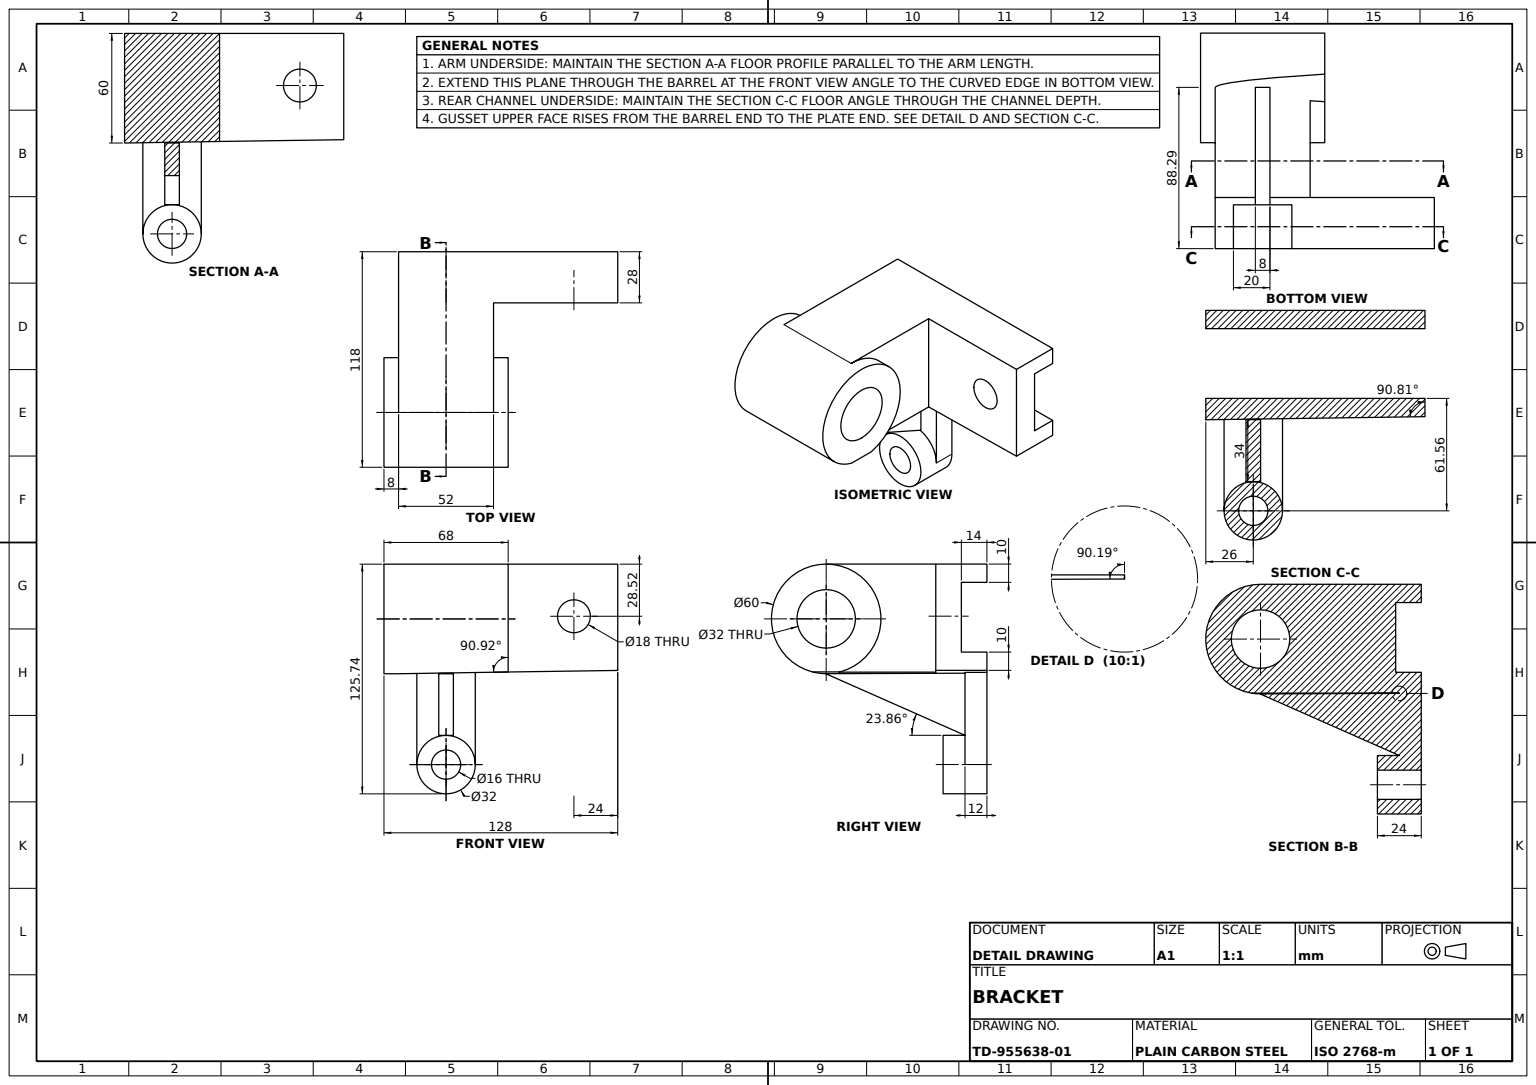
ISO-10303-21;
HEADER;
FILE_DESCRIPTION((''),'2;1');
FILE_NAME('','',(''),(''),'','','');
FILE_SCHEMA(('AUTOMOTIVE_DESIGN'));
ENDSEC;
DATA;
#1=APPLICATION_CONTEXT('');
#2=PRODUCT_CONTEXT('',#1,'mechanical');
#3=PRODUCT('','','',(#2));
#4=PRODUCT_DEFINITION_FORMATION('','',#3);
#5=PRODUCT_DEFINITION_CONTEXT('',#1,'design');
#6=PRODUCT_DEFINITION('','',#4,#5);
#7=PRODUCT_DEFINITION_SHAPE('','',#6);
#8=(LENGTH_UNIT()NAMED_UNIT(*)SI_UNIT(.MILLI.,.METRE.));
#9=(NAMED_UNIT(*)PLANE_ANGLE_UNIT()SI_UNIT($,.RADIAN.));
#10=(NAMED_UNIT(*)SI_UNIT($,.STERADIAN.)SOLID_ANGLE_UNIT());
#11=UNCERTAINTY_MEASURE_WITH_UNIT(LENGTH_MEASURE(1.E-05),#8,'distance_accuracy_value','');
#12=(GEOMETRIC_REPRESENTATION_CONTEXT(3)GLOBAL_UNCERTAINTY_ASSIGNED_CONTEXT((#11))GLOBAL_UNIT_ASSIGNED_CONTEXT((#8,#9,#10))REPRESENTATION_CONTEXT('',''));
#13=CARTESIAN_POINT('',(113.,31.478195,14.));
#14=VERTEX_POINT('',#13);
#15=CARTESIAN_POINT('',(113.,31.478195,28.));
#16=VERTEX_POINT('',#15);
#17=CARTESIAN_POINT('',(113.,31.478195,-100.));
#18=DIRECTION('',(0.,0.,1.));
#19=VECTOR('',#18,1000.);
#20=LINE('',#17,#19);
#21=EDGE_CURVE('',#14,#16,#20,.T.);
#22=ORIENTED_EDGE('',*,*,#21,.T.);
#23=CARTESIAN_POINT('',(95.,31.478195,28.));
#24=VERTEX_POINT('',#23);
#25=CARTESIAN_POINT('',(104.,31.478195,28.));
#26=DIRECTION('',(1.,0.,0.));
#27=AXIS2_PLACEMENT_3D('',#25,#18,#26);
#28=CIRCLE('',#27,9.);
#29=EDGE_CURVE('',#16,#24,#28,.T.);
#30=ORIENTED_EDGE('',*,*,#29,.T.);
#31=CARTESIAN_POINT('',(95.,31.478195,14.));
#32=VERTEX_POINT('',#31);
#33=CARTESIAN_POINT('',(95.,31.478195,-100.));
#34=LINE('',#33,#19);
#35=EDGE_CURVE('',#32,#24,#34,.T.);
#36=ORIENTED_EDGE('',*,*,#35,.F.);
#37=CARTESIAN_POINT('',(104.,31.478195,14.));
#38=AXIS2_PLACEMENT_3D('',#37,#18,#26);
#39=CIRCLE('',#38,9.);
#40=EDGE_CURVE('',#14,#32,#39,.T.);
#41=ORIENTED_EDGE('',*,*,#40,.F.);
#42=EDGE_LOOP('',(#22,#30,#36,#41));
#43=FACE_OUTER_BOUND('',#42,.T.);
#44=CARTESIAN_POINT('',(104.,31.478195,-100.));
#45=AXIS2_PLACEMENT_3D('',#44,#18,#26);
#46=CYLINDRICAL_SURFACE('',#45,9.);
#47=ADVANCED_FACE('',(#43),#46,.F.);
#48=CARTESIAN_POINT('',(50.,-49.744681,24.));
#49=VERTEX_POINT('',#48);
#50=CARTESIAN_POINT('',(50.,-49.744681,12.));
#51=VERTEX_POINT('',#50);
#52=DIRECTION('',(0.,0.,-1.));
#53=VECTOR('',#52,1000.);
#54=LINE('',#50,#53);
#55=EDGE_CURVE('',#49,#51,#54,.T.);
#56=ORIENTED_EDGE('',*,*,#55,.T.);
#57=CARTESIAN_POINT('',(34.,-33.744681,12.));
#58=VERTEX_POINT('',#57);
#59=CARTESIAN_POINT('',(34.,-49.744681,12.));
#60=AXIS2_PLACEMENT_3D('',#59,#18,#26);
#61=CIRCLE('',#60,16.);
#62=EDGE_CURVE('',#51,#58,#61,.T.);
#63=ORIENTED_EDGE('',*,*,#62,.T.);
#64=CARTESIAN_POINT('',(18.,-49.744681,12.));
#65=VERTEX_POINT('',#64);
#66=EDGE_CURVE('',#58,#65,#61,.T.);
#67=ORIENTED_EDGE('',*,*,#66,.T.);
#68=CARTESIAN_POINT('',(18.,-49.744681,24.));
#69=VERTEX_POINT('',#68);
#70=LINE('',#64,#53);
#71=EDGE_CURVE('',#69,#65,#70,.T.);
#72=ORIENTED_EDGE('',*,*,#71,.F.);
#73=CARTESIAN_POINT('',(34.,-49.744681,24.));
#74=AXIS2_PLACEMENT_3D('',#73,#18,#26);
#75=CIRCLE('',#74,16.);
#76=EDGE_CURVE('',#49,#69,#75,.T.);
#77=ORIENTED_EDGE('',*,*,#76,.F.);
#78=EDGE_LOOP('',(#56,#63,#67,#72,#77));
#79=FACE_OUTER_BOUND('',#78,.T.);
#80=DIRECTION('',(-1.,0.,0.));
#81=AXIS2_PLACEMENT_3D('',#59,#52,#80);
#82=CYLINDRICAL_SURFACE('',#81,16.);
#83=ADVANCED_FACE('',(#79),#82,.T.);
#84=CARTESIAN_POINT('',(8.,0.113475,28.));
#85=VERTEX_POINT('',#84);
#86=CARTESIAN_POINT('',(60.,0.851064,28.));
#87=VERTEX_POINT('',#86);
#88=CARTESIAN_POINT('',(0.,0.,28.));
#89=DIRECTION('',(0.999899417,0.01418297,0.));
#90=VECTOR('',#89,1000.);
#91=LINE('',#88,#90);
#92=EDGE_CURVE('',#85,#87,#91,.T.);
#93=ORIENTED_EDGE('',*,*,#92,.T.);
#94=CARTESIAN_POINT('',(60.,0.835934,28.));
#95=VERTEX_POINT('',#94);
#96=CARTESIAN_POINT('',(60.,60.,28.));
#97=DIRECTION('',(0.,1.,0.));
#98=VECTOR('',#97,1000.);
#99=LINE('',#96,#98);
#100=EDGE_CURVE('',#95,#87,#99,.T.);
#101=ORIENTED_EDGE('',*,*,#100,.F.);
#102=CARTESIAN_POINT('',(8.,0.,28.));
#103=VERTEX_POINT('',#102);
#104=CARTESIAN_POINT('',(68.,0.964539,28.));
#105=DIRECTION('',(0.999870812,0.016073573,0.));
#106=VECTOR('',#105,1000.);
#107=LINE('',#104,#106);
#108=EDGE_CURVE('',#103,#95,#107,.T.);
#109=ORIENTED_EDGE('',*,*,#108,.F.);
#110=LINE('',#102,#98);
#111=EDGE_CURVE('',#103,#85,#110,.T.);
#112=ORIENTED_EDGE('',*,*,#111,.T.);
#113=EDGE_LOOP('',(#93,#101,#109,#112));
#114=FACE_OUTER_BOUND('',#113,.T.);
#115=CARTESIAN_POINT('',(68.,0.,28.));
#116=AXIS2_PLACEMENT_3D('',#115,#52,#80);
#117=PLANE('',#116);
#118=ADVANCED_FACE('',(#114),#117,.T.);
#119=CARTESIAN_POINT('',(8.,11.815603,0.));
#120=VERTEX_POINT('',#119);
#121=CARTESIAN_POINT('',(8.,0.113475,0.));
#122=VERTEX_POINT('',#121);
#123=DIRECTION('',(0.,-1.,0.));
#124=VECTOR('',#123,1000.);
#125=LINE('',#119,#124);
#126=EDGE_CURVE('',#120,#122,#125,.T.);
#127=ORIENTED_EDGE('',*,*,#126,.T.);
#128=LINE('',#84,#19);
#129=EDGE_CURVE('',#122,#85,#128,.T.);
#130=ORIENTED_EDGE('',*,*,#129,.T.);
#131=ORIENTED_EDGE('',*,*,#111,.F.);
#132=CARTESIAN_POINT('',(8.,0.,88.));
#133=VERTEX_POINT('',#132);
#134=CARTESIAN_POINT('',(8.,0.,0.));
#135=LINE('',#134,#19);
#136=EDGE_CURVE('',#103,#133,#135,.T.);
#137=ORIENTED_EDGE('',*,*,#136,.T.);
#138=CARTESIAN_POINT('',(8.,60.,88.));
#139=VERTEX_POINT('',#138);
#140=CARTESIAN_POINT('',(8.,30.,88.));
#141=AXIS2_PLACEMENT_3D('',#140,#26,#123);
#142=CIRCLE('',#141,30.);
#143=EDGE_CURVE('',#133,#139,#142,.T.);
#144=ORIENTED_EDGE('',*,*,#143,.T.);
#145=CARTESIAN_POINT('',(8.,60.,0.));
#146=VERTEX_POINT('',#145);
#147=LINE('',#145,#53);
#148=EDGE_CURVE('',#139,#146,#147,.T.);
#149=ORIENTED_EDGE('',*,*,#148,.T.);
#150=CARTESIAN_POINT('',(8.,50.,0.));
#151=VERTEX_POINT('',#150);
#152=LINE('',#145,#124);
#153=EDGE_CURVE('',#146,#151,#152,.T.);
#154=ORIENTED_EDGE('',*,*,#153,.T.);
#155=CARTESIAN_POINT('',(8.,50.,14.));
#156=VERTEX_POINT('',#155);
#157=LINE('',#150,#19);
#158=EDGE_CURVE('',#151,#156,#157,.T.);
#159=ORIENTED_EDGE('',*,*,#158,.T.);
#160=CARTESIAN_POINT('',(8.,11.815603,14.));
#161=VERTEX_POINT('',#160);
#162=LINE('',#155,#124);
#163=EDGE_CURVE('',#156,#161,#162,.T.);
#164=ORIENTED_EDGE('',*,*,#163,.T.);
#165=LINE('',#160,#53);
#166=EDGE_CURVE('',#161,#120,#165,.T.);
#167=ORIENTED_EDGE('',*,*,#166,.T.);
#168=EDGE_LOOP('',(#127,#130,#131,#137,#144,#149,#154,#159,#164,#167));
#169=FACE_OUTER_BOUND('',#168,.T.);
#170=AXIS2_PLACEMENT_3D('',#140,#80,#123);
#171=PLANE('',#170);
#172=ADVANCED_FACE('',(#169),#171,.T.);
#173=CARTESIAN_POINT('',(0.,60.,88.));
#174=VERTEX_POINT('',#173);
#175=VECTOR('',#26,1000.);
#176=LINE('',#173,#175);
#177=EDGE_CURVE('',#174,#139,#176,.T.);
#178=ORIENTED_EDGE('',*,*,#177,.F.);
#179=CARTESIAN_POINT('',(0.,0.,88.));
#180=VERTEX_POINT('',#179);
#181=CARTESIAN_POINT('',(0.,30.,88.));
#182=AXIS2_PLACEMENT_3D('',#181,#26,#97);
#183=CIRCLE('',#182,30.);
#184=EDGE_CURVE('',#174,#180,#183,.T.);
#185=ORIENTED_EDGE('',*,*,#184,.T.);
#186=LINE('',#179,#175);
#187=EDGE_CURVE('',#180,#133,#186,.T.);
#188=ORIENTED_EDGE('',*,*,#187,.T.);
#189=CARTESIAN_POINT('',(68.,0.964539,95.545993));
#190=VERTEX_POINT('',#189);
#191=CARTESIAN_POINT('',(28.108187,0.323252,93.07845));
#192=CARTESIAN_POINT('',(8.,0.,90.549513));
#193=(BOUNDED_CURVE()B_SPLINE_CURVE(3,(#189,#191,#192,#132),.UNSPECIFIED.,.F.,.F.)B_SPLINE_CURVE_WITH_KNOTS((4,4),(2.887328708,3.141592654),.UNSPECIFIED.)CURVE()GEOMETRIC_REPRESENTATION_ITEM()RATIONAL_B_SPLINE_CURVE((1.,0.99461974,0.99461974,1.))REPRESENTATION_ITEM(''));
#194=EDGE_CURVE('',#190,#133,#193,.T.);
#195=ORIENTED_EDGE('',*,*,#194,.F.);
#196=CARTESIAN_POINT('',(68.,60.,88.));
#197=VERTEX_POINT('',#196);
#198=CARTESIAN_POINT('',(68.,30.,88.));
#199=AXIS2_PLACEMENT_3D('',#198,#26,#97);
#200=CIRCLE('',#199,30.);
#201=EDGE_CURVE('',#197,#190,#200,.T.);
#202=ORIENTED_EDGE('',*,*,#201,.F.);
#203=CARTESIAN_POINT('',(60.,60.,88.));
#204=VERTEX_POINT('',#203);
#205=EDGE_CURVE('',#204,#197,#176,.T.);
#206=ORIENTED_EDGE('',*,*,#205,.F.);
#207=VECTOR('',#80,1000.);
#208=LINE('',#196,#207);
#209=EDGE_CURVE('',#204,#139,#208,.T.);
#210=ORIENTED_EDGE('',*,*,#209,.T.);
#211=EDGE_LOOP('',(#178,#185,#188,#195,#202,#206,#210));
#212=FACE_OUTER_BOUND('',#211,.T.);
#213=CYLINDRICAL_SURFACE('',#182,30.);
#214=ADVANCED_FACE('',(#212),#213,.T.);
#215=CARTESIAN_POINT('',(18.,0.255319,12.));
#216=VERTEX_POINT('',#215);
#217=CARTESIAN_POINT('',(18.,0.255319,0.));
#218=VERTEX_POINT('',#217);
#219=LINE('',#215,#53);
#220=EDGE_CURVE('',#216,#218,#219,.T.);
#221=ORIENTED_EDGE('',*,*,#220,.T.);
#222=CARTESIAN_POINT('',(18.,-49.744681,0.));
#223=VERTEX_POINT('',#222);
#224=LINE('',#217,#98);
#225=EDGE_CURVE('',#223,#218,#224,.T.);
#226=ORIENTED_EDGE('',*,*,#225,.F.);
#227=EDGE_CURVE('',#65,#223,#70,.T.);
#228=ORIENTED_EDGE('',*,*,#227,.F.);
#229=LINE('',#215,#98);
#230=EDGE_CURVE('',#65,#216,#229,.T.);
#231=ORIENTED_EDGE('',*,*,#230,.T.);
#232=EDGE_LOOP('',(#221,#226,#228,#231));
#233=FACE_OUTER_BOUND('',#232,.T.);
#234=AXIS2_PLACEMENT_3D('',#215,#80,#123);
#235=PLANE('',#234);
#236=ADVANCED_FACE('',(#233),#235,.T.);
#237=CARTESIAN_POINT('',(42.,-49.744681,0.));
#238=VERTEX_POINT('',#237);
#239=CARTESIAN_POINT('',(42.,-49.744681,24.));
#240=VERTEX_POINT('',#239);
#241=LINE('',#237,#19);
#242=EDGE_CURVE('',#238,#240,#241,.T.);
#243=ORIENTED_EDGE('',*,*,#242,.F.);
#244=CARTESIAN_POINT('',(26.,-49.744681,0.));
#245=VERTEX_POINT('',#244);
#246=CARTESIAN_POINT('',(34.,-49.744681,0.));
#247=AXIS2_PLACEMENT_3D('',#246,#18,#26);
#248=CIRCLE('',#247,8.);
#249=EDGE_CURVE('',#245,#238,#248,.T.);
#250=ORIENTED_EDGE('',*,*,#249,.F.);
#251=CARTESIAN_POINT('',(26.,-49.744681,24.));
#252=VERTEX_POINT('',#251);
#253=LINE('',#244,#19);
#254=EDGE_CURVE('',#245,#252,#253,.T.);
#255=ORIENTED_EDGE('',*,*,#254,.T.);
#256=CIRCLE('',#74,8.);
#257=EDGE_CURVE('',#252,#240,#256,.T.);
#258=ORIENTED_EDGE('',*,*,#257,.T.);
#259=EDGE_LOOP('',(#243,#250,#255,#258));
#260=FACE_OUTER_BOUND('',#259,.T.);
#261=CYLINDRICAL_SURFACE('',#247,8.);
#262=ADVANCED_FACE('',(#260),#261,.F.);
#263=CARTESIAN_POINT('',(0.,46.,88.));
#264=VERTEX_POINT('',#263);
#265=CARTESIAN_POINT('',(68.,46.,88.));
#266=VERTEX_POINT('',#265);
#267=LINE('',#263,#175);
#268=EDGE_CURVE('',#264,#266,#267,.T.);
#269=ORIENTED_EDGE('',*,*,#268,.F.);
#270=CARTESIAN_POINT('',(0.,14.,88.));
#271=VERTEX_POINT('',#270);
#272=CIRCLE('',#182,16.);
#273=EDGE_CURVE('',#271,#264,#272,.T.);
#274=ORIENTED_EDGE('',*,*,#273,.F.);
#275=CARTESIAN_POINT('',(68.,14.,88.));
#276=VERTEX_POINT('',#275);
#277=LINE('',#270,#175);
#278=EDGE_CURVE('',#271,#276,#277,.T.);
#279=ORIENTED_EDGE('',*,*,#278,.T.);
#280=CIRCLE('',#199,16.);
#281=EDGE_CURVE('',#276,#266,#280,.T.);
#282=ORIENTED_EDGE('',*,*,#281,.T.);
#283=EDGE_LOOP('',(#269,#274,#279,#282));
#284=FACE_OUTER_BOUND('',#283,.T.);
#285=CYLINDRICAL_SURFACE('',#182,16.);
#286=ADVANCED_FACE('',(#284),#285,.F.);
#287=CARTESIAN_POINT('',(50.,0.70922,0.));
#288=VERTEX_POINT('',#287);
#289=CARTESIAN_POINT('',(50.,-49.744681,0.));
#290=VERTEX_POINT('',#289);
#291=LINE('',#289,#124);
#292=EDGE_CURVE('',#288,#290,#291,.T.);
#293=ORIENTED_EDGE('',*,*,#292,.T.);
#294=AXIS2_PLACEMENT_3D('',#246,#52,#80);
#295=CIRCLE('',#294,16.);
#296=EDGE_CURVE('',#290,#223,#295,.T.);
#297=ORIENTED_EDGE('',*,*,#296,.T.);
#298=ORIENTED_EDGE('',*,*,#225,.T.);
#299=CARTESIAN_POINT('',(0.,0.,0.));
#300=LINE('',#299,#90);
#301=EDGE_CURVE('',#122,#218,#300,.T.);
#302=ORIENTED_EDGE('',*,*,#301,.F.);
#303=ORIENTED_EDGE('',*,*,#126,.F.);
#304=CARTESIAN_POINT('',(128.,11.815603,0.));
#305=VERTEX_POINT('',#304);
#306=CARTESIAN_POINT('',(0.,11.815603,0.));
#307=LINE('',#306,#175);
#308=EDGE_CURVE('',#120,#305,#307,.T.);
#309=ORIENTED_EDGE('',*,*,#308,.T.);
#310=CARTESIAN_POINT('',(128.,1.815603,0.));
#311=VERTEX_POINT('',#310);
#312=LINE('',#310,#98);
#313=EDGE_CURVE('',#311,#305,#312,.T.);
#314=ORIENTED_EDGE('',*,*,#313,.F.);
#315=EDGE_CURVE('',#288,#311,#300,.T.);
#316=ORIENTED_EDGE('',*,*,#315,.F.);
#317=EDGE_LOOP('',(#293,#297,#298,#302,#303,#309,#314,#316));
#318=FACE_OUTER_BOUND('',#317,.T.);
#319=ORIENTED_EDGE('',*,*,#249,.T.);
#320=EDGE_CURVE('',#238,#245,#248,.T.);
#321=ORIENTED_EDGE('',*,*,#320,.T.);
#322=EDGE_LOOP('',(#319,#321));
#323=FACE_BOUND('',#322,.T.);
#324=AXIS2_PLACEMENT_3D('',#299,#52,#80);
#325=PLANE('',#324);
#326=ADVANCED_FACE('',(#318,#323),#325,.T.);
#327=EDGE_CURVE('',#240,#252,#256,.T.);
#328=ORIENTED_EDGE('',*,*,#327,.T.);
#329=ORIENTED_EDGE('',*,*,#254,.F.);
#330=ORIENTED_EDGE('',*,*,#320,.F.);
#331=ORIENTED_EDGE('',*,*,#242,.T.);
#332=EDGE_LOOP('',(#328,#329,#330,#331));
#333=FACE_OUTER_BOUND('',#332,.T.);
#334=ADVANCED_FACE('',(#333),#261,.F.);
#335=ORIENTED_EDGE('',*,*,#177,.T.);
#336=ORIENTED_EDGE('',*,*,#143,.F.);
#337=ORIENTED_EDGE('',*,*,#187,.F.);
#338=EDGE_CURVE('',#180,#174,#183,.T.);
#339=ORIENTED_EDGE('',*,*,#338,.T.);
#340=EDGE_LOOP('',(#335,#336,#337,#339));
#341=FACE_OUTER_BOUND('',#340,.T.);
#342=ADVANCED_FACE('',(#341),#213,.T.);
#343=EDGE_CURVE('',#51,#290,#54,.T.);
#344=ORIENTED_EDGE('',*,*,#343,.T.);
#345=ORIENTED_EDGE('',*,*,#292,.F.);
#346=CARTESIAN_POINT('',(50.,0.70922,12.));
#347=VERTEX_POINT('',#346);
#348=LINE('',#346,#53);
#349=EDGE_CURVE('',#347,#288,#348,.T.);
#350=ORIENTED_EDGE('',*,*,#349,.F.);
#351=LINE('',#50,#124);
#352=EDGE_CURVE('',#347,#51,#351,.T.);
#353=ORIENTED_EDGE('',*,*,#352,.T.);
#354=EDGE_LOOP('',(#344,#345,#350,#353));
#355=FACE_OUTER_BOUND('',#354,.T.);
#356=AXIS2_PLACEMENT_3D('',#50,#26,#97);
#357=PLANE('',#356);
#358=ADVANCED_FACE('',(#355),#357,.T.);
#359=CARTESIAN_POINT('',(38.,0.,88.292467));
#360=VERTEX_POINT('',#359);
#361=CARTESIAN_POINT('',(38.,-33.744681,12.));
#362=VERTEX_POINT('',#361);
#363=DIRECTION('',(0.,-0.404505371,-0.914535622));
#364=VECTOR('',#363,1000.);
#365=LINE('',#361,#364);
#366=EDGE_CURVE('',#360,#362,#365,.T.);
#367=ORIENTED_EDGE('',*,*,#366,.F.);
#368=CARTESIAN_POINT('',(30.,0.,88.292467));
#369=VERTEX_POINT('',#368);
#370=LINE('',#368,#175);
#371=EDGE_CURVE('',#369,#360,#370,.T.);
#372=ORIENTED_EDGE('',*,*,#371,.F.);
#373=CARTESIAN_POINT('',(30.,-33.744681,12.));
#374=VERTEX_POINT('',#373);
#375=LINE('',#373,#364);
#376=EDGE_CURVE('',#369,#374,#375,.T.);
#377=ORIENTED_EDGE('',*,*,#376,.T.);
#378=LINE('',#373,#175);
#379=EDGE_CURVE('',#374,#58,#378,.T.);
#380=ORIENTED_EDGE('',*,*,#379,.T.);
#381=LINE('',#57,#207);
#382=EDGE_CURVE('',#362,#58,#381,.T.);
#383=ORIENTED_EDGE('',*,*,#382,.F.);
#384=EDGE_LOOP('',(#367,#372,#377,#380,#383));
#385=FACE_OUTER_BOUND('',#384,.T.);
#386=DIRECTION('',(0.,-0.914535622,0.404505371));
#387=AXIS2_PLACEMENT_3D('',#373,#386,#363);
#388=PLANE('',#387);
#389=ADVANCED_FACE('',(#385),#388,.T.);
#390=ORIENTED_EDGE('',*,*,#21,.F.);
#391=EDGE_CURVE('',#32,#14,#39,.T.);
#392=ORIENTED_EDGE('',*,*,#391,.F.);
#393=ORIENTED_EDGE('',*,*,#35,.T.);
#394=EDGE_CURVE('',#24,#16,#28,.T.);
#395=ORIENTED_EDGE('',*,*,#394,.T.);
#396=EDGE_LOOP('',(#390,#392,#393,#395));
#397=FACE_OUTER_BOUND('',#396,.T.);
#398=ADVANCED_FACE('',(#397),#46,.F.);
#399=ORIENTED_EDGE('',*,*,#371,.T.);
#400=CARTESIAN_POINT('',(38.,0.255319,12.));
#401=VERTEX_POINT('',#400);
#402=DIRECTION('',(0.,-0.003346565,0.9999944));
#403=VECTOR('',#402,1000.);
#404=LINE('',#359,#403);
#405=EDGE_CURVE('',#401,#360,#404,.T.);
#406=ORIENTED_EDGE('',*,*,#405,.F.);
#407=CARTESIAN_POINT('',(30.,0.255319,12.));
#408=VERTEX_POINT('',#407);
#409=LINE('',#407,#175);
#410=EDGE_CURVE('',#408,#401,#409,.T.);
#411=ORIENTED_EDGE('',*,*,#410,.F.);
#412=LINE('',#368,#403);
#413=EDGE_CURVE('',#408,#369,#412,.T.);
#414=ORIENTED_EDGE('',*,*,#413,.T.);
#415=EDGE_LOOP('',(#399,#406,#411,#414));
#416=FACE_OUTER_BOUND('',#415,.T.);
#417=DIRECTION('',(0.,0.9999944,0.003346565));
#418=AXIS2_PLACEMENT_3D('',#368,#417,#402);
#419=PLANE('',#418);
#420=ADVANCED_FACE('',(#416),#419,.T.);
#421=CARTESIAN_POINT('',(128.,60.,28.));
#422=VERTEX_POINT('',#421);
#423=CARTESIAN_POINT('',(128.,60.,0.));
#424=VERTEX_POINT('',#423);
#425=LINE('',#421,#53);
#426=EDGE_CURVE('',#422,#424,#425,.T.);
#427=ORIENTED_EDGE('',*,*,#426,.F.);
#428=CARTESIAN_POINT('',(128.,1.815603,28.));
#429=VERTEX_POINT('',#428);
#430=LINE('',#428,#98);
#431=EDGE_CURVE('',#429,#422,#430,.T.);
#432=ORIENTED_EDGE('',*,*,#431,.F.);
#433=LINE('',#428,#53);
#434=EDGE_CURVE('',#429,#311,#433,.T.);
#435=ORIENTED_EDGE('',*,*,#434,.T.);
#436=ORIENTED_EDGE('',*,*,#313,.T.);
#437=CARTESIAN_POINT('',(128.,11.815603,14.));
#438=VERTEX_POINT('',#437);
#439=LINE('',#304,#53);
#440=EDGE_CURVE('',#438,#305,#439,.T.);
#441=ORIENTED_EDGE('',*,*,#440,.F.);
#442=CARTESIAN_POINT('',(128.,50.,14.));
#443=VERTEX_POINT('',#442);
#444=CARTESIAN_POINT('',(128.,0.,14.));
#445=LINE('',#444,#124);
#446=EDGE_CURVE('',#443,#438,#445,.T.);
#447=ORIENTED_EDGE('',*,*,#446,.F.);
#448=CARTESIAN_POINT('',(128.,50.,0.));
#449=VERTEX_POINT('',#448);
#450=LINE('',#448,#19);
#451=EDGE_CURVE('',#449,#443,#450,.T.);
#452=ORIENTED_EDGE('',*,*,#451,.F.);
#453=EDGE_CURVE('',#449,#424,#312,.T.);
#454=ORIENTED_EDGE('',*,*,#453,.T.);
#455=EDGE_LOOP('',(#427,#432,#435,#436,#441,#447,#452,#454));
#456=FACE_OUTER_BOUND('',#455,.T.);
#457=AXIS2_PLACEMENT_3D('',#428,#80,#18);
#458=PLANE('',#457);
#459=ADVANCED_FACE('',(#456),#458,.F.);
#460=ORIENTED_EDGE('',*,*,#100,.T.);
#461=VERTEX_POINT('',#96);
#462=EDGE_CURVE('',#87,#461,#99,.T.);
#463=ORIENTED_EDGE('',*,*,#462,.T.);
#464=LINE('',#203,#19);
#465=EDGE_CURVE('',#461,#204,#464,.T.);
#466=ORIENTED_EDGE('',*,*,#465,.T.);
#467=CARTESIAN_POINT('',(60.,0.835934,80.967416));
#468=VERTEX_POINT('',#467);
#469=CARTESIAN_POINT('',(60.,30.,88.));
#470=AXIS2_PLACEMENT_3D('',#469,#80,#97);
#471=CIRCLE('',#470,30.);
#472=EDGE_CURVE('',#204,#468,#471,.T.);
#473=ORIENTED_EDGE('',*,*,#472,.T.);
#474=CARTESIAN_POINT('',(60.,0.835934,88.));
#475=LINE('',#474,#19);
#476=EDGE_CURVE('',#95,#468,#475,.T.);
#477=ORIENTED_EDGE('',*,*,#476,.F.);
#478=EDGE_LOOP('',(#460,#463,#466,#473,#477));
#479=FACE_OUTER_BOUND('',#478,.T.);
#480=AXIS2_PLACEMENT_3D('',#469,#26,#97);
#481=PLANE('',#480);
#482=ADVANCED_FACE('',(#479),#481,.T.);
#483=ORIENTED_EDGE('',*,*,#184,.F.);
#484=ORIENTED_EDGE('',*,*,#338,.F.);
#485=EDGE_LOOP('',(#483,#484));
#486=FACE_OUTER_BOUND('',#485,.T.);
#487=ORIENTED_EDGE('',*,*,#273,.T.);
#488=EDGE_CURVE('',#264,#271,#272,.T.);
#489=ORIENTED_EDGE('',*,*,#488,.T.);
#490=EDGE_LOOP('',(#487,#489));
#491=FACE_BOUND('',#490,.T.);
#492=CARTESIAN_POINT('',(0.,60.,28.));
#493=AXIS2_PLACEMENT_3D('',#492,#26,#97);
#494=PLANE('',#493);
#495=ADVANCED_FACE('',(#486,#491),#494,.F.);
#496=ORIENTED_EDGE('',*,*,#379,.F.);
#497=LINE('',#407,#98);
#498=EDGE_CURVE('',#374,#408,#497,.T.);
#499=ORIENTED_EDGE('',*,*,#498,.T.);
#500=ORIENTED_EDGE('',*,*,#410,.T.);
#501=LINE('',#400,#98);
#502=EDGE_CURVE('',#362,#401,#501,.T.);
#503=ORIENTED_EDGE('',*,*,#502,.F.);
#504=ORIENTED_EDGE('',*,*,#382,.T.);
#505=ORIENTED_EDGE('',*,*,#62,.F.);
#506=ORIENTED_EDGE('',*,*,#352,.F.);
#507=LINE('',#346,#90);
#508=EDGE_CURVE('',#216,#347,#507,.T.);
#509=ORIENTED_EDGE('',*,*,#508,.F.);
#510=ORIENTED_EDGE('',*,*,#230,.F.);
#511=ORIENTED_EDGE('',*,*,#66,.F.);
#512=EDGE_LOOP('',(#496,#499,#500,#503,#504,#505,#506,#509,#510,#511));
#513=FACE_OUTER_BOUND('',#512,.T.);
#514=PLANE('',#81);
#515=ADVANCED_FACE('',(#513),#514,.F.);
#516=ORIENTED_EDGE('',*,*,#257,.F.);
#517=ORIENTED_EDGE('',*,*,#327,.F.);
#518=EDGE_LOOP('',(#516,#517));
#519=FACE_BOUND('',#518,.T.);
#520=EDGE_CURVE('',#69,#49,#75,.T.);
#521=ORIENTED_EDGE('',*,*,#520,.T.);
#522=ORIENTED_EDGE('',*,*,#76,.T.);
#523=EDGE_LOOP('',(#521,#522));
#524=FACE_OUTER_BOUND('',#523,.T.);
#525=PLANE('',#74);
#526=ADVANCED_FACE('',(#519,#524),#525,.T.);
#527=ORIENTED_EDGE('',*,*,#451,.T.);
#528=CARTESIAN_POINT('',(0.,50.,14.));
#529=LINE('',#528,#175);
#530=EDGE_CURVE('',#156,#443,#529,.T.);
#531=ORIENTED_EDGE('',*,*,#530,.F.);
#532=ORIENTED_EDGE('',*,*,#158,.F.);
#533=CARTESIAN_POINT('',(0.,50.,0.));
#534=LINE('',#533,#175);
#535=EDGE_CURVE('',#151,#449,#534,.T.);
#536=ORIENTED_EDGE('',*,*,#535,.T.);
#537=EDGE_LOOP('',(#527,#531,#532,#536));
#538=FACE_OUTER_BOUND('',#537,.T.);
#539=AXIS2_PLACEMENT_3D('',#533,#97,#18);
#540=PLANE('',#539);
#541=ADVANCED_FACE('',(#538),#540,.F.);
#542=ORIENTED_EDGE('',*,*,#153,.F.);
#543=LINE('',#423,#207);
#544=EDGE_CURVE('',#424,#146,#543,.T.);
#545=ORIENTED_EDGE('',*,*,#544,.F.);
#546=ORIENTED_EDGE('',*,*,#453,.F.);
#547=ORIENTED_EDGE('',*,*,#535,.F.);
#548=EDGE_LOOP('',(#542,#545,#546,#547));
#549=FACE_OUTER_BOUND('',#548,.T.);
#550=ADVANCED_FACE('',(#549),#325,.T.);
#551=ORIENTED_EDGE('',*,*,#136,.F.);
#552=ORIENTED_EDGE('',*,*,#108,.T.);
#553=ORIENTED_EDGE('',*,*,#476,.T.);
#554=CARTESIAN_POINT('',(68.,0.964539,80.454007));
#555=VERTEX_POINT('',#554);
#556=CARTESIAN_POINT('',(62.572722,0.877292,80.795904));
#557=CARTESIAN_POINT('',(65.239458,0.920162,80.624763));
#558=(BOUNDED_CURVE()B_SPLINE_CURVE(3,(#467,#556,#557,#554),.UNSPECIFIED.,.F.,.T.)B_SPLINE_CURVE_WITH_KNOTS((4,4),(3.378214018,3.3958566),.UNSPECIFIED.)CURVE()GEOMETRIC_REPRESENTATION_ITEM()RATIONAL_B_SPLINE_CURVE((1.,0.999974062,0.999974062,1.))REPRESENTATION_ITEM(''));
#559=EDGE_CURVE('',#468,#555,#558,.T.);
#560=ORIENTED_EDGE('',*,*,#559,.T.);
#561=CARTESIAN_POINT('',(68.,0.964539,128.));
#562=LINE('',#561,#53);
#563=EDGE_CURVE('',#190,#555,#562,.T.);
#564=ORIENTED_EDGE('',*,*,#563,.F.);
#565=ORIENTED_EDGE('',*,*,#194,.T.);
#566=EDGE_LOOP('',(#551,#552,#553,#560,#564,#565));
#567=FACE_OUTER_BOUND('',#566,.T.);
#568=DIRECTION('',(-0.016073573,0.999870812,0.));
#569=DIRECTION('',(-0.999870812,-0.016073573,0.));
#570=AXIS2_PLACEMENT_3D('',#561,#568,#569);
#571=PLANE('',#570);
#572=ADVANCED_FACE('',(#567),#571,.F.);
#573=ORIENTED_EDGE('',*,*,#278,.F.);
#574=ORIENTED_EDGE('',*,*,#488,.F.);
#575=ORIENTED_EDGE('',*,*,#268,.T.);
#576=EDGE_CURVE('',#266,#276,#280,.T.);
#577=ORIENTED_EDGE('',*,*,#576,.T.);
#578=EDGE_LOOP('',(#573,#574,#575,#577));
#579=FACE_OUTER_BOUND('',#578,.T.);
#580=ADVANCED_FACE('',(#579),#285,.F.);
#581=CARTESIAN_POINT('',(0.,11.815603,14.));
#582=LINE('',#581,#175);
#583=EDGE_CURVE('',#161,#438,#582,.T.);
#584=ORIENTED_EDGE('',*,*,#583,.T.);
#585=ORIENTED_EDGE('',*,*,#440,.T.);
#586=ORIENTED_EDGE('',*,*,#308,.F.);
#587=ORIENTED_EDGE('',*,*,#166,.F.);
#588=EDGE_LOOP('',(#584,#585,#586,#587));
#589=FACE_OUTER_BOUND('',#588,.T.);
#590=AXIS2_PLACEMENT_3D('',#306,#123,#52);
#591=PLANE('',#590);
#592=ADVANCED_FACE('',(#589),#591,.F.);
#593=ORIENTED_EDGE('',*,*,#394,.F.);
#594=ORIENTED_EDGE('',*,*,#29,.F.);
#595=EDGE_LOOP('',(#593,#594));
#596=FACE_BOUND('',#595,.T.);
#597=LINE('',#421,#207);
#598=EDGE_CURVE('',#422,#461,#597,.T.);
#599=ORIENTED_EDGE('',*,*,#598,.T.);
#600=ORIENTED_EDGE('',*,*,#462,.F.);
#601=EDGE_CURVE('',#87,#429,#91,.T.);
#602=ORIENTED_EDGE('',*,*,#601,.T.);
#603=ORIENTED_EDGE('',*,*,#431,.T.);
#604=EDGE_LOOP('',(#599,#600,#602,#603));
#605=FACE_OUTER_BOUND('',#604,.T.);
#606=AXIS2_PLACEMENT_3D('',#88,#52,#80);
#607=PLANE('',#606);
#608=ADVANCED_FACE('',(#596,#605),#607,.F.);
#609=ORIENTED_EDGE('',*,*,#520,.F.);
#610=ORIENTED_EDGE('',*,*,#71,.T.);
#611=ORIENTED_EDGE('',*,*,#227,.T.);
#612=ORIENTED_EDGE('',*,*,#296,.F.);
#613=ORIENTED_EDGE('',*,*,#343,.F.);
#614=ORIENTED_EDGE('',*,*,#55,.F.);
#615=EDGE_LOOP('',(#609,#610,#611,#612,#613,#614));
#616=FACE_OUTER_BOUND('',#615,.T.);
#617=ADVANCED_FACE('',(#616),#82,.T.);
#618=ORIENTED_EDGE('',*,*,#446,.T.);
#619=ORIENTED_EDGE('',*,*,#583,.F.);
#620=ORIENTED_EDGE('',*,*,#163,.F.);
#621=ORIENTED_EDGE('',*,*,#530,.T.);
#622=EDGE_LOOP('',(#618,#619,#620,#621));
#623=FACE_OUTER_BOUND('',#622,.T.);
#624=ORIENTED_EDGE('',*,*,#391,.T.);
#625=ORIENTED_EDGE('',*,*,#40,.T.);
#626=EDGE_LOOP('',(#624,#625));
#627=FACE_BOUND('',#626,.T.);
#628=CARTESIAN_POINT('',(0.,0.,14.));
#629=AXIS2_PLACEMENT_3D('',#628,#18,#26);
#630=PLANE('',#629);
#631=ADVANCED_FACE('',(#623,#627),#630,.F.);
#632=ORIENTED_EDGE('',*,*,#576,.F.);
#633=ORIENTED_EDGE('',*,*,#281,.F.);
#634=EDGE_LOOP('',(#632,#633));
#635=FACE_BOUND('',#634,.T.);
#636=ORIENTED_EDGE('',*,*,#563,.T.);
#637=EDGE_CURVE('',#555,#197,#200,.T.);
#638=ORIENTED_EDGE('',*,*,#637,.T.);
#639=ORIENTED_EDGE('',*,*,#201,.T.);
#640=EDGE_LOOP('',(#636,#638,#639));
#641=FACE_OUTER_BOUND('',#640,.T.);
#642=CARTESIAN_POINT('',(68.,0.,0.));
#643=AXIS2_PLACEMENT_3D('',#642,#26,#97);
#644=PLANE('',#643);
#645=ADVANCED_FACE('',(#635,#641),#644,.T.);
#646=ORIENTED_EDGE('',*,*,#209,.F.);
#647=ORIENTED_EDGE('',*,*,#465,.F.);
#648=ORIENTED_EDGE('',*,*,#598,.F.);
#649=ORIENTED_EDGE('',*,*,#426,.T.);
#650=ORIENTED_EDGE('',*,*,#544,.T.);
#651=ORIENTED_EDGE('',*,*,#148,.F.);
#652=EDGE_LOOP('',(#646,#647,#648,#649,#650,#651));
#653=FACE_OUTER_BOUND('',#652,.T.);
#654=AXIS2_PLACEMENT_3D('',#421,#123,#26);
#655=PLANE('',#654);
#656=ADVANCED_FACE('',(#653),#655,.F.);
#657=ORIENTED_EDGE('',*,*,#366,.T.);
#658=ORIENTED_EDGE('',*,*,#502,.T.);
#659=ORIENTED_EDGE('',*,*,#405,.T.);
#660=EDGE_LOOP('',(#657,#658,#659));
#661=FACE_OUTER_BOUND('',#660,.T.);
#662=CARTESIAN_POINT('',(38.,0.,0.));
#663=AXIS2_PLACEMENT_3D('',#662,#26,#97);
#664=PLANE('',#663);
#665=ADVANCED_FACE('',(#661),#664,.T.);
#666=ORIENTED_EDGE('',*,*,#413,.F.);
#667=ORIENTED_EDGE('',*,*,#498,.F.);
#668=ORIENTED_EDGE('',*,*,#376,.F.);
#669=EDGE_LOOP('',(#666,#667,#668));
#670=FACE_OUTER_BOUND('',#669,.T.);
#671=CARTESIAN_POINT('',(30.,0.,0.));
#672=AXIS2_PLACEMENT_3D('',#671,#80,#123);
#673=PLANE('',#672);
#674=ADVANCED_FACE('',(#670),#673,.T.);
#675=ORIENTED_EDGE('',*,*,#637,.F.);
#676=ORIENTED_EDGE('',*,*,#559,.F.);
#677=ORIENTED_EDGE('',*,*,#472,.F.);
#678=ORIENTED_EDGE('',*,*,#205,.T.);
#679=EDGE_LOOP('',(#675,#676,#677,#678));
#680=FACE_OUTER_BOUND('',#679,.T.);
#681=ADVANCED_FACE('',(#680),#213,.T.);
#682=ORIENTED_EDGE('',*,*,#508,.T.);
#683=ORIENTED_EDGE('',*,*,#349,.T.);
#684=ORIENTED_EDGE('',*,*,#315,.T.);
#685=ORIENTED_EDGE('',*,*,#434,.F.);
#686=ORIENTED_EDGE('',*,*,#601,.F.);
#687=ORIENTED_EDGE('',*,*,#92,.F.);
#688=ORIENTED_EDGE('',*,*,#129,.F.);
#689=ORIENTED_EDGE('',*,*,#301,.T.);
#690=ORIENTED_EDGE('',*,*,#220,.F.);
#691=EDGE_LOOP('',(#682,#683,#684,#685,#686,#687,#688,#689,#690));
#692=FACE_OUTER_BOUND('',#691,.T.);
#693=DIRECTION('',(-0.01418297,0.999899417,0.));
#694=DIRECTION('',(-0.999899417,-0.01418297,0.));
#695=AXIS2_PLACEMENT_3D('',#88,#693,#694);
#696=PLANE('',#695);
#697=ADVANCED_FACE('',(#692),#696,.F.);
#698=CLOSED_SHELL('',(#47,#83,#118,#172,#214,#236,#262,#286,#326,#334,#342,#358,#389,#398,#420,#459,#482,#495,#515,#526,#541,#550,#572,#580,#592,#608,#617,#631,#645,#656,#665,#674,#681,#697));
#699=MANIFOLD_SOLID_BREP('',#698);
#700=ADVANCED_BREP_SHAPE_REPRESENTATION('',(#699),#12);
#701=SHAPE_DEFINITION_REPRESENTATION(#7,#700);
ENDSEC;
END-ISO-10303-21;
